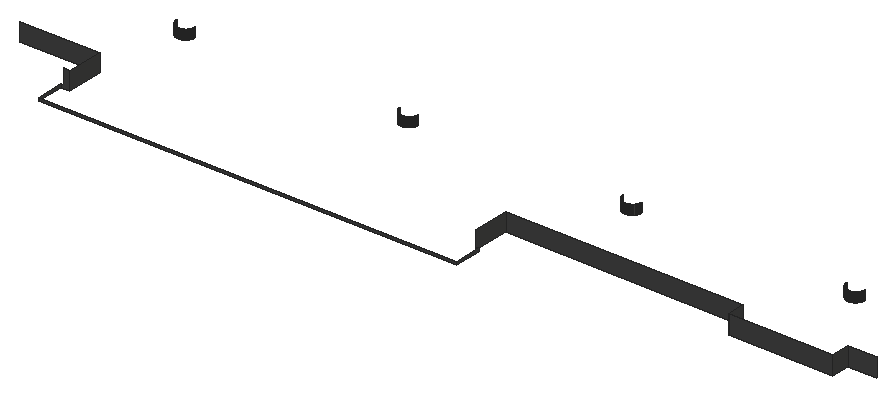
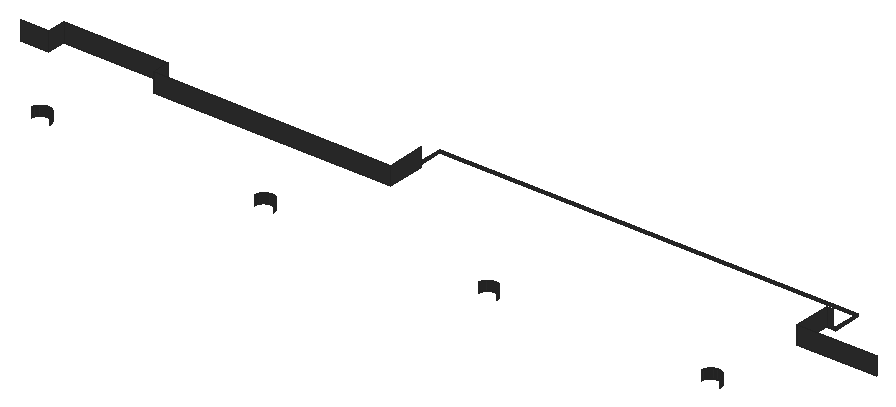
# SketchUp Ruby script. Lengths in inches.
U = 1.inch
M = Sketchup.active_model
def pt(a) = Geom::Point3d.new(a.map { |v| v * U })
def face(e, loops, mat)
  f = e.add_face(loops[0].map { |a| pt(a) })
  loops[1..].each { |l| e.add_face(l.map { |a| pt(a) }).erase! }
  f.material = f.back_material = mat if mat
  f
end
# faces: each face lists its corners as indices into pts; further lists are holes
def faces(e, pts, list, mat = nil) = list.each { |f| face(e, (f[0].is_a?(Array) ? f : [f]).map { |l| l.map { |i| pts[i] } }, mat) }
# xy, xz, yz: faces in a plane at the given z, y or x. An outline is a flat list of corners, or four numbers for a rectangle; further outlines are holes
def ring(l) = l.size == 4 ? [[l[0], l[1]], [l[2], l[1]], [l[2], l[3]], [l[0], l[3]]] : l.each_slice(2).to_a
def flat(e, list, mat, &to3) = list.each { |f| face(e, (f[0].is_a?(Array) ? f : [f]).map { |l| ring(l).map { |u, v| to3.(u, v) } }, mat) }
def xy(e, z, list, mat = nil) = flat(e, list, mat) { |x, y| [x, y, z] }
def xz(e, y, list, mat = nil) = flat(e, list, mat) { |x, z| [x, y, z] }
def yz(e, x, list, mat = nil) = flat(e, list, mat) { |y, z| [x, y, z] }
def lines(e, pts, list) = list.each { |a, b| e.add_line(pt(pts[a]), pt(pts[b])) }
# prism: a flat outline (further loops are holes) pulled along v
def prism(e, loops, v, mat = nil)
  f = face(e, loops, mat); d = Geom::Vector3d.new(v.map { |x| x * U })
  f.pushpull(f.normal.samedirection?(d) ? d.length : -d.length)
end
def box(e, o, s, mat = nil) = prism(e, [[o, [o[0] + s[0], o[1], o[2]], [o[0] + s[0], o[1] + s[1], o[2]], [o[0], o[1] + s[1], o[2]]]], [0, 0, s[2]], mat)
def at(x, y, z, deg = 0) = Geom::Transformation.translation(pt([x, y, z])) * Geom::Transformation.rotation(ORIGIN, Z_AXIS, deg.degrees)
def axes(o, x, y, z) = Geom::Transformation.new([*x, 0, *y, 0, *z, 0, *pt(o).to_a, 1])
def part(name) = M.definitions.add(name)
# library, detail: a bought-in or finely detailed component or shape, given as its bounding box
def library(name, o, s) = part(name).tap { |d| box(d.entities, o, s) }
def detail(e, o, s) = box(e.add_group.entities, o, s)
def put(e, d, t, mat = nil) = e.add_instance(d, t).tap { |i| i.material = mat if mat }
def group(e, t, mat = nil) = e.add_group.tap { |g| g.transformation = t; g.material = mat if mat }.entities
root = M.entities
M.materials.add("1448 AP 8253 RAVEN SONG").color = [64, 64, 63]
xz(root,174,[[31.93,372,167.89,373]],"1448 AP 8253 RAVEN SONG")
xz(root,183,[[31.93,372,31.93,373,32.96,373,32.96,378,35.02,378,35.02,372],[166.86,372,167.89,373]],"1448 AP 8253 RAVEN SONG")
xz(root,189,[[244.11,372,278.1,378]],"1448 AP 8253 RAVEN SONG")
xz(root,195,[[9.27,372,35.02,378],[166.86,372,244.11,378],[278.1,372,287.37,378]],"1448 AP 8253 RAVEN SONG")
xz(root,221.5,[[39.29,372,39.37,375],[39.37,372,39.45,375],[39.45,372,39.53,375],[39.53,372,39.61,375],[111.87,372,111.95,375],
  [111.95,372,112.03,375],[112.03,372,112.11,375],[112.11,372,112.1875,375],[184.45,372,184.53,375],[184.53,372,184.61,375],
  [184.61,372,184.6875,375],[184.6875,372,184.77,375],[257.03,372,257.11,375],[257.11,372,257.19,375],[257.19,372,257.27,375],
  [257.27,372,257.35,375]],"1448 AP 8253 RAVEN SONG")
yz(root,31.93,[[174,372,183,373]],"1448 AP 8253 RAVEN SONG")
yz(root,35.02,[[183,372,195,378]],"1448 AP 8253 RAVEN SONG")
yz(root,36.45,[[224.34,372,224.42,375]],"1448 AP 8253 RAVEN SONG")
yz(root,42.45,[[224.34,372,224.42,375]],"1448 AP 8253 RAVEN SONG")
yz(root,109.03,[[224.34,372,224.42,375]],"1448 AP 8253 RAVEN SONG")
yz(root,115.03,[[224.34,372,224.42,375]],"1448 AP 8253 RAVEN SONG")
yz(root,166.86,[[183,372,195,378]],"1448 AP 8253 RAVEN SONG")
yz(root,167.89,[[174,372,183,373]],"1448 AP 8253 RAVEN SONG")
yz(root,181.61,[[224.34,372,224.42,375]],"1448 AP 8253 RAVEN SONG")
yz(root,187.61,[[224.34,372,224.42,375],[224.42,372,224.5,375]],"1448 AP 8253 RAVEN SONG")
yz(root,244.11,[[189,372,195,378]],"1448 AP 8253 RAVEN SONG")
yz(root,254.19,[[224.34,372,224.42,375],[224.42,372,224.5,375]],"1448 AP 8253 RAVEN SONG")
yz(root,260.1875,[[224.34,372,224.42,375]],"1448 AP 8253 RAVEN SONG")
yz(root,278.1,[[189,372,195,378]],"1448 AP 8253 RAVEN SONG")
p = [[38.98,221.54,372],[38.9,221.55,372],[38.9,221.55,375],[38.98,221.54,375],[39.06,221.53,372],[39.06,221.53,375],
  [39.21,221.51,372],[39.14,221.52,372],[39.14,221.52,375],[39.21,221.51,375],[39.29,221.5,372],[39.29,221.5,375],
  [39.69,221.51,372],[39.61,221.5,372],[39.61,221.5,375],[39.69,221.51,375],[39.76,221.52,372],[39.76,221.52,375],
  [39.84,221.53,372],[39.84,221.53,375],[39.92,221.54,372],[39.92,221.54,375],[40,221.55,372],[40,221.55,375],
  [111.5625,221.54,372],[111.48,221.55,372],[111.48,221.55,375],[111.5625,221.54,375],[111.72,221.52,372],[111.64,221.53,372],
  [111.64,221.53,375],[111.72,221.52,375],[111.79,221.51,372],[111.79,221.51,375],[111.87,221.5,372],[111.87,221.5,375],
  [112.27,221.51,372],[112.1875,221.5,372],[112.1875,221.5,375],[112.27,221.51,375],[112.34,221.52,372],[112.34,221.52,375],
  [112.42,221.53,372],[112.42,221.53,375],[112.5,221.54,372],[112.5,221.54,375],[112.58,221.55,372],[112.58,221.55,375],
  [184.22,221.53,372],[184.14,221.54,372],[184.14,221.54,375],[184.22,221.53,375],[184.0625,221.55,372],[184.0625,221.55,375],
  [184.3,221.52,372],[184.3,221.52,375],[184.375,221.51,372],[184.375,221.51,375],[184.45,221.5,372],[184.45,221.5,375],
  [184.85,221.51,372],[184.77,221.5,372],[184.77,221.5,375],[184.85,221.51,375],[184.92,221.52,372],[184.92,221.52,375],
  [185,221.53,372],[185,221.53,375],[185.08,221.54,372],[185.08,221.54,375],[185.16,221.55,372],[185.16,221.55,375],
  [256.72,221.54,372],[256.64,221.55,372],[256.64,221.55,375],[256.72,221.54,375],[256.8,221.53,372],[256.8,221.53,375],
  [256.875,221.52,372],[256.875,221.52,375],[256.95,221.51,372],[256.95,221.51,375],[257.03,221.5,372],[257.03,221.5,375],
  [257.43,221.51,372],[257.35,221.5,372],[257.35,221.5,375],[257.43,221.51,375],[257.5,221.52,372],[257.5,221.52,375],
  [257.58,221.53,372],[257.58,221.53,375],[257.66,221.54,372],[257.66,221.54,375],[257.74,221.55,372],[257.74,221.55,375],
  [38.52,221.65,372],[38.45,221.67,372],[38.45,221.67,375],[38.52,221.65,375],[38.6,221.625,372],[38.6,221.625,375],
  [38.67,221.6,372],[38.67,221.6,375],[38.83,221.57,372],[38.75,221.58,372],[38.75,221.58,375],[38.83,221.57,375],
  [40.07,221.57,372],[40.07,221.57,375],[40.15,221.58,372],[40.15,221.58,375],[40.23,221.6,372],[40.23,221.6,375],
  [40.3,221.625,372],[40.3,221.625,375],[40.38,221.65,372],[40.38,221.65,375],[40.45,221.67,372],[40.45,221.67,375],
  [111.1,221.65,372],[111.03,221.67,372],[111.03,221.67,375],[111.1,221.65,375],[111.18,221.625,372],[111.18,221.625,375],
  [111.25,221.6,372],[111.25,221.6,375],[111.41,221.57,372],[111.33,221.58,372],[111.33,221.58,375],[111.41,221.57,375],
  [112.65,221.57,372],[112.65,221.57,375],[112.73,221.58,372],[112.73,221.58,375],[112.81,221.6,372],[112.81,221.6,375],
  [112.88,221.625,372],[112.88,221.625,375],[112.96,221.65,372],[112.96,221.65,375],[113.03,221.67,372],[113.03,221.67,375],
  [183.68,221.65,372],[183.61,221.67,372],[183.61,221.67,375],[183.68,221.65,375],[183.76,221.625,372],[183.76,221.625,375],
  [183.91,221.58,372],[183.83,221.6,372],[183.83,221.6,375],[183.91,221.58,375],[183.99,221.57,372],[183.99,221.57,375],
  [185.23,221.57,372],[185.23,221.57,375],[185.31,221.58,372],[185.31,221.58,375],[185.39,221.6,372],[185.39,221.6,375],
  [185.46,221.625,372],[185.46,221.625,375],[185.54,221.65,372],[185.54,221.65,375],[185.61,221.67,372],[185.61,221.67,375],
  [256.26,221.65,372],[256.1875,221.67,372],[256.1875,221.67,375],[256.26,221.65,375],[256.41,221.6,372],[256.34,221.625,372],
  [256.34,221.625,375],[256.41,221.6,375],[256.49,221.58,372],[256.49,221.58,375],[256.57,221.57,372],[256.57,221.57,375],
  [257.8125,221.57,372],[257.8125,221.57,375],[257.89,221.58,372],[257.89,221.58,375],[257.97,221.6,372],[257.97,221.6,375],
  [258.04,221.625,372],[258.04,221.625,375],[258.12,221.65,372],[258.12,221.65,375],[258.19,221.67,372],[258.19,221.67,375],
  [38.3,221.73,372],[38.23,221.76,372],[38.23,221.76,375],[38.3,221.73,375],[38.375,221.7,372],[38.375,221.7,375],
  [40.53,221.7,372],[40.53,221.7,375],[40.6,221.73,372],[40.6,221.73,375],[40.67,221.76,372],[40.67,221.76,375],
  [110.88,221.73,372],[110.81,221.76,372],[110.81,221.76,375],[110.88,221.73,375],[110.95,221.7,372],[110.95,221.7,375],
  [113.11,221.7,372],[113.11,221.7,375],[113.18,221.73,372],[113.18,221.73,375],[113.25,221.76,372],[113.25,221.76,375],
  [183.46,221.73,372],[183.39,221.76,372],[183.39,221.76,375],[183.46,221.73,375],[183.53,221.7,372],[183.53,221.7,375],
  [185.69,221.7,372],[185.69,221.7,375],[185.76,221.73,372],[185.76,221.73,375],[185.83,221.76,372],[185.83,221.76,375],
  [256.11,221.7,372],[256.04,221.73,372],[256.04,221.73,375],[256.11,221.7,375],[255.97,221.76,372],[255.97,221.76,375],
  [258.27,221.7,372],[258.27,221.7,375],[258.34,221.73,372],[258.34,221.73,375],[258.41,221.76,372],[258.41,221.76,375],
  [38.09,221.83,372],[38.02,221.86,372],[38.02,221.86,375],[38.09,221.83,375],[38.16,221.79,372],[38.16,221.79,375],
  [40.74,221.79,372],[40.74,221.79,375],[40.8125,221.83,372],[40.8125,221.83,375],[40.88,221.86,372],[40.88,221.86,375],
  [110.67,221.83,372],[110.6,221.86,372],[110.6,221.86,375],[110.67,221.83,375],[110.74,221.79,372],[110.74,221.79,375],
  [113.32,221.79,372],[113.32,221.79,375],[113.39,221.83,372],[113.39,221.83,375],[113.46,221.86,372],[113.46,221.86,375],
  [183.32,221.79,372],[183.25,221.83,372],[183.25,221.83,375],[183.32,221.79,375],[183.18,221.86,372],[183.18,221.86,375],
  [185.9,221.79,372],[185.9,221.79,375],[185.97,221.83,372],[185.97,221.83,375],[186.04,221.86,372],[186.04,221.86,375],
  [255.9,221.79,372],[255.83,221.83,372],[255.83,221.83,375],[255.9,221.79,375],[255.76,221.86,372],[255.76,221.86,375],
  [258.48,221.79,372],[258.48,221.79,375],[258.55,221.83,372],[258.55,221.83,375],[258.62,221.86,372],[258.62,221.86,375],
  [37.88,221.94,372],[37.82,221.98,372],[37.82,221.98,375],[37.88,221.94,375],[37.95,221.9,372],[37.95,221.9,375],
  [40.95,221.9,372],[40.95,221.9,375],[41.02,221.94,372],[41.02,221.94,375],[41.08,221.98,372],[41.08,221.98,375],
  [110.46,221.94,372],[110.4,221.98,372],[110.4,221.98,375],[110.46,221.94,375],[110.53,221.9,372],[110.53,221.9,375],
  [113.53,221.9,372],[113.53,221.9,375],[113.6,221.94,372],[113.6,221.94,375],[113.66,221.98,372],[113.66,221.98,375],
  [183.11,221.9,372],[183.04,221.94,372],[183.04,221.94,375],[183.11,221.9,375],[182.98,221.98,372],[182.98,221.98,375],
  [186.11,221.9,372],[186.11,221.9,375],[186.18,221.94,372],[186.18,221.94,375],[186.24,221.98,372],[186.24,221.98,375],
  [255.69,221.9,372],[255.62,221.94,372],[255.62,221.94,375],[255.69,221.9,375],[255.56,221.98,372],[255.56,221.98,375],
  [258.69,221.9,372],[258.69,221.9,375],[258.76,221.94,372],[258.76,221.94,375],[258.82,221.98,372],[258.82,221.98,375],
  [37.75,222.03,372],[37.6875,222.07,372],[37.6875,222.07,375],[37.75,222.03,375],[41.15,222.03,372],[41.15,222.03,375],
  [41.21,222.07,372],[41.21,222.07,375],[110.33,222.03,372],[110.33,222.03,375],[110.27,222.07,372],[110.27,222.07,375],
  [113.73,222.03,372],[113.73,222.03,375],[113.79,222.07,372],[113.79,222.07,375],[182.91,222.03,372],[182.85,222.07,372],
  [182.85,222.07,375],[182.91,222.03,375],[186.31,222.03,372],[186.31,222.03,375],[186.375,222.07,372],[186.375,222.07,375],
  [255.49,222.03,372],[255.43,222.07,372],[255.43,222.07,375],[255.49,222.03,375],[258.89,222.03,372],[258.89,222.03,375],
  [258.95,222.07,372],[258.95,222.07,375],[37.625,222.12,372],[37.625,222.12,375],[37.5625,222.17,372],[37.5625,222.17,375],
  [41.28,222.12,372],[41.28,222.12,375],[41.34,222.17,372],[41.34,222.17,375],[110.2,222.12,372],[110.14,222.17,372],
  [110.14,222.17,375],[110.2,222.12,375],[113.86,222.12,372],[113.86,222.12,375],[113.92,222.17,372],[113.92,222.17,375],
  [182.78,222.12,372],[182.72,222.17,372],[182.72,222.17,375],[182.78,222.12,375],[186.4375,222.12,372],[186.4375,222.12,375],
  [186.5,222.17,372],[186.5,222.17,375],[255.36,222.12,372],[255.3,222.17,372],[255.3,222.17,375],[255.36,222.12,375],
  [259.02,222.12,372],[259.02,222.12,375],[259.08,222.17,372],[259.08,222.17,375],[37.5,222.22,372],[37.44,222.27,372],
  [37.44,222.27,375],[37.5,222.22,375],[41.4,222.22,372],[41.4,222.22,375],[41.46,222.27,372],[41.46,222.27,375],
  [110.08,222.22,372],[110.02,222.27,372],[110.02,222.27,375],[110.08,222.22,375],[113.98,222.22,372],[113.98,222.22,375],
  [114.04,222.27,372],[114.04,222.27,375],[182.66,222.22,372],[182.6,222.27,372],[182.6,222.27,375],[182.66,222.22,375],
  [186.56,222.22,372],[186.56,222.22,375],[186.62,222.27,372],[186.62,222.27,375],[255.24,222.22,372],[255.24,222.22,375],
  [255.18,222.27,372],[255.18,222.27,375],[259.14,222.22,372],[259.14,222.22,375],[259.2,222.27,372],[259.2,222.27,375],
  [37.38,222.32,372],[37.33,222.38,372],[37.33,222.38,375],[37.38,222.32,375],[41.52,222.32,372],[41.52,222.32,375],
  [41.57,222.38,372],[41.57,222.38,375],[109.96,222.32,372],[109.91,222.38,372],[109.91,222.38,375],[109.96,222.32,375],
  [114.1,222.32,372],[114.1,222.32,375],[114.15,222.38,372],[114.15,222.38,375],[182.54,222.32,372],[182.54,222.32,375],
  [182.49,222.38,372],[182.49,222.38,375],[186.68,222.32,372],[186.68,222.32,375],[186.73,222.38,372],[186.73,222.38,375],
  [255.125,222.32,372],[255.125,222.32,375],[255.07,222.38,372],[255.07,222.38,375],[259.26,222.32,372],[259.26,222.32,375],
  [259.3125,222.38,372],[259.3125,222.38,375],[37.27,222.43,372],[37.22,222.49,372],[37.22,222.49,375],[37.27,222.43,375],
  [41.625,222.43,372],[41.625,222.43,375],[41.68,222.49,372],[41.68,222.49,375],[109.85,222.43,372],[109.8,222.49,372],
  [109.8,222.49,375],[109.85,222.43,375],[114.21,222.43,372],[114.21,222.43,375],[114.26,222.49,372],[114.26,222.49,375],
  [182.43,222.43,372],[182.43,222.43,375],[182.38,222.49,372],[182.38,222.49,375],[186.79,222.43,372],[186.79,222.43,375],
  [186.84,222.49,372],[186.84,222.49,375],[255.01,222.43,372],[255.01,222.43,375],[254.96,222.49,372],[254.96,222.49,375],
  [259.37,222.43,372],[259.37,222.43,375],[259.42,222.49,372],[259.42,222.49,375],[37.17,222.55,372],[37.17,222.55,375],
  [41.73,222.55,372],[41.73,222.55,375],[109.75,222.55,372],[109.75,222.55,375],[114.3125,222.55,372],[114.3125,222.55,375],
  [182.33,222.55,372],[182.33,222.55,375],[186.89,222.55,372],[186.89,222.55,375],[254.91,222.55,372],[254.91,222.55,375],
  [259.47,222.55,372],[259.47,222.55,375],[37.12,222.61,372],[37.12,222.61,375],[37.07,222.67,372],[37.07,222.67,375],
  [41.78,222.61,372],[41.78,222.61,375],[41.83,222.67,372],[41.83,222.67,375],[109.7,222.61,372],[109.65,222.67,372],
  [109.65,222.67,375],[109.7,222.61,375],[114.36,222.61,372],[114.36,222.61,375],[114.41,222.67,372],[114.41,222.67,375],
  [182.28,222.61,372],[182.23,222.67,372],[182.23,222.67,375],[182.28,222.61,375],[186.94,222.61,372],[186.94,222.61,375],
  [186.99,222.67,372],[186.99,222.67,375],[254.86,222.61,372],[254.81,222.67,372],[254.81,222.67,375],[254.86,222.61,375],
  [259.52,222.61,372],[259.52,222.61,375],[259.57,222.67,372],[259.57,222.67,375],[37.02,222.74,372],[37.02,222.74,375],
  [36.98,222.8,372],[36.98,222.8,375],[41.88,222.74,372],[41.88,222.74,375],[41.92,222.8,372],[41.92,222.8,375],
  [109.6,222.74,372],[109.6,222.74,375],[109.56,222.8,372],[109.56,222.8,375],[114.46,222.74,372],[114.46,222.74,375],
  [114.5,222.8,372],[114.5,222.8,375],[182.18,222.74,372],[182.14,222.8,372],[182.14,222.8,375],[182.18,222.74,375],
  [187.04,222.74,372],[187.04,222.74,375],[187.08,222.8,372],[187.08,222.8,375],[254.76,222.74,372],[254.72,222.8,372],
  [254.72,222.8,375],[254.76,222.74,375],[259.62,222.74,372],[259.62,222.74,375],[259.66,222.8,372],[259.66,222.8,375],
  [36.93,222.87,372],[36.93,222.87,375],[41.97,222.87,372],[41.97,222.87,375],[109.51,222.87,372],[109.51,222.87,375],
  [114.55,222.87,372],[114.55,222.87,375],[182.09,222.87,372],[182.09,222.87,375],[187.125,222.87,372],[187.125,222.87,375],
  [254.67,222.87,372],[254.67,222.87,375],[259.71,222.87,372],[259.71,222.87,375],[36.89,222.93,372],[36.89,222.93,375],
  [36.85,223,372],[36.85,223,375],[42.01,222.93,372],[42.01,222.93,375],[42.05,223,372],[42.05,223,375],
  [109.47,222.93,372],[109.43,223,372],[109.43,223,375],[109.47,222.93,375],[114.59,222.93,372],[114.59,222.93,375],
  [114.63,223,372],[114.63,223,375],[182.05,222.93,372],[182.01,223,372],[182.01,223,375],[182.05,222.93,375],
  [187.17,222.93,372],[187.17,222.93,375],[187.21,223,372],[187.21,223,375],[254.63,222.93,372],[254.63,222.93,375],
  [254.59,223,372],[254.59,223,375],[259.75,222.93,372],[259.75,222.93,375],[259.79,223,372],[259.79,223,375],
  [36.8125,223.07,372],[36.8125,223.07,375],[42.09,223.07,372],[42.09,223.07,375],[109.39,223.07,372],[109.39,223.07,375],
  [114.67,223.07,372],[114.67,223.07,375],[181.97,223.07,372],[181.97,223.07,375],[187.25,223.07,372],[187.25,223.07,375],
  [254.55,223.07,372],[254.55,223.07,375],[259.83,223.07,372],[259.83,223.07,375],[36.78,223.14,372],[36.74,223.21,372],
  [36.74,223.21,375],[36.78,223.14,375],[42.125,223.14,372],[42.125,223.14,375],[42.16,223.21,372],[42.16,223.21,375],
  [109.36,223.14,372],[109.32,223.21,372],[109.32,223.21,375],[109.36,223.14,375],[114.7,223.14,372],[114.7,223.14,375],
  [114.74,223.21,372],[114.74,223.21,375],[181.9375,223.14,372],[181.9375,223.14,375],[181.9,223.21,372],[181.9,223.21,375],
  [187.28,223.14,372],[187.28,223.14,375],[187.32,223.21,372],[187.32,223.21,375],[254.52,223.14,372],[254.52,223.14,375],
  [254.48,223.21,372],[254.48,223.21,375],[259.86,223.14,372],[259.86,223.14,375],[259.9,223.21,372],[259.9,223.21,375],
  [36.71,223.28,372],[36.71,223.28,375],[42.19,223.28,372],[42.19,223.28,375],[109.29,223.28,372],[109.29,223.28,375],
  [114.77,223.28,372],[114.77,223.28,375],[181.87,223.28,372],[181.87,223.28,375],[187.35,223.28,372],[187.35,223.28,375],
  [254.45,223.28,372],[254.45,223.28,375],[259.93,223.28,372],[259.93,223.28,375],[36.68,223.35,372],[36.68,223.35,375],
  [42.22,223.35,372],[42.22,223.35,375],[109.26,223.35,372],[109.26,223.35,375],[114.8,223.35,372],[114.8,223.35,375],
  [181.84,223.35,372],[181.84,223.35,375],[187.38,223.35,372],[187.38,223.35,375],[254.42,223.35,372],[254.42,223.35,375],
  [259.96,223.35,372],[259.96,223.35,375],[36.65,223.42,372],[36.65,223.42,375],[36.62,223.5,372],[36.62,223.5,375],
  [42.25,223.42,372],[42.25,223.42,375],[42.28,223.5,372],[42.28,223.5,375],[109.23,223.42,372],[109.23,223.42,375],
  [109.2,223.5,372],[109.2,223.5,375],[114.83,223.42,372],[114.83,223.42,375],[114.86,223.5,372],[114.86,223.5,375],
  [181.81,223.42,372],[181.81,223.42,375],[181.78,223.5,372],[181.78,223.5,375],[187.41,223.42,372],[187.41,223.42,375],
  [187.4375,223.5,372],[187.4375,223.5,375],[254.39,223.42,372],[254.39,223.42,375],[254.36,223.5,372],[254.36,223.5,375],
  [259.99,223.42,372],[259.99,223.42,375],[260.02,223.5,372],[260.02,223.5,375],[36.6,223.57,372],[36.6,223.57,375],
  [42.3,223.57,372],[42.3,223.57,375],[109.18,223.57,372],[109.18,223.57,375],[114.88,223.57,372],[114.88,223.57,375],
  [181.76,223.57,372],[181.76,223.57,375],[187.46,223.57,372],[187.46,223.57,375],[254.34,223.57,372],[254.34,223.57,375],
  [260.04,223.57,372],[260.04,223.57,375],[36.57,223.65,372],[36.57,223.65,375],[36.55,223.72,372],[36.55,223.72,375],
  [42.33,223.65,372],[42.33,223.65,375],[42.35,223.72,372],[42.35,223.72,375],[109.15,223.65,372],[109.13,223.72,372],
  [109.13,223.72,375],[109.15,223.65,375],[114.91,223.65,372],[114.91,223.65,375],[114.93,223.72,372],[114.93,223.72,375],
  [181.73,223.65,372],[181.73,223.65,375],[181.71,223.72,372],[181.71,223.72,375],[187.49,223.65,372],[187.49,223.65,375],
  [187.51,223.72,372],[187.51,223.72,375],[254.3125,223.65,372],[254.3125,223.65,375],[254.29,223.72,372],[254.29,223.72,375],
  [260.07,223.65,372],[260.07,223.65,375],[260.09,223.72,372],[260.09,223.72,375],[36.53,223.8,372],[36.53,223.8,375],
  [42.37,223.8,372],[42.37,223.8,375],[109.11,223.8,372],[109.11,223.8,375],[114.95,223.8,372],[114.95,223.8,375],
  [181.69,223.8,372],[181.69,223.8,375],[187.53,223.8,372],[187.53,223.8,375],[254.27,223.8,372],[254.27,223.8,375],
  [260.11,223.8,372],[260.11,223.8,375],[36.52,223.875,372],[36.52,223.875,375],[42.38,223.875,372],[42.38,223.875,375],
  [109.1,223.875,372],[109.1,223.875,375],[114.96,223.875,372],[114.96,223.875,375],[181.68,223.875,372],[181.68,223.875,375],
  [187.54,223.875,372],[187.54,223.875,375],[254.26,223.875,372],[254.26,223.875,375],[260.125,223.875,372],[260.125,223.875,375],
  [36.5,223.95,372],[36.5,223.95,375],[42.4,223.95,372],[42.4,223.95,375],[109.08,223.95,372],[109.08,223.95,375],
  [114.98,223.95,372],[114.98,223.95,375],[181.66,223.95,372],[181.66,223.95,375],[187.56,223.95,372],[187.56,223.95,375],
  [254.24,223.95,372],[254.24,223.95,375],[260.14,223.95,372],[260.14,223.95,375],[36.49,224.03,372],[36.49,224.03,375],
  [36.48,224.11,372],[36.48,224.11,375],[42.41,224.03,372],[42.41,224.03,375],[42.42,224.11,372],[42.42,224.11,375],
  [109.07,224.03,372],[109.07,224.03,375],[109.06,224.11,372],[109.06,224.11,375],[114.99,224.03,372],[114.99,224.03,375],
  [115,224.11,372],[115,224.11,375],[181.65,224.03,372],[181.65,224.03,375],[181.64,224.11,372],[181.64,224.11,375],
  [187.57,224.03,372],[187.57,224.03,375],[187.58,224.11,372],[187.58,224.11,375],[254.23,224.03,372],[254.23,224.03,375],
  [254.22,224.11,372],[254.22,224.11,375],[260.15,224.03,372],[260.15,224.03,375],[260.16,224.11,372],[260.16,224.11,375],
  [36.47,224.1875,372],[36.47,224.1875,375],[42.43,224.1875,372],[42.43,224.1875,375],[109.05,224.1875,372],[109.05,224.1875,375],
  [115.01,224.1875,372],[115.01,224.1875,375],[181.625,224.1875,372],[181.625,224.1875,375],[187.59,224.1875,372],[187.59,224.1875,375],
  [254.21,224.1875,372],[254.21,224.1875,375],[260.17,224.1875,372],[260.17,224.1875,375],[36.46,224.26,372],[36.46,224.26,375],
  [42.44,224.26,372],[42.44,224.26,375],[109.04,224.26,372],[109.04,224.26,375],[115.02,224.26,372],[115.02,224.26,375],
  [181.62,224.26,372],[181.62,224.26,375],[187.6,224.26,372],[187.6,224.26,375],[254.2,224.26,372],[254.2,224.26,375],
  [260.18,224.26,372],[260.18,224.26,375],[36.45,224.34,372],[36.45,224.34,375],[42.45,224.34,372],[42.45,224.34,375],
  [109.03,224.34,372],[109.03,224.34,375],[115.03,224.34,372],[115.03,224.34,375],[181.61,224.34,372],[181.61,224.34,375],
  [187.61,224.34,372],[187.61,224.34,375],[254.19,224.34,372],[254.19,224.34,375],[260.1875,224.34,372],[260.1875,224.34,375],
  [260.19,224.5,372],[260.1875,224.42,372],[260.1875,224.42,375],[260.19,224.5,375]]
faces(root,p,[[0,1,2,3],[4,0,3,5],[6,7,8,9],[7,4,5,8],[10,6,9,11],[12,13,14,15],[16,12,15,17],[18,16,17,19],
  [20,18,19,21],[22,20,21,23],[24,25,26,27],[28,29,30,31],[29,24,27,30],[32,28,31,33],[34,32,33,35],[36,37,38,39],
  [40,36,39,41],[42,40,41,43],[44,42,43,45],[46,44,45,47],[48,49,50,51],[49,52,53,50],[54,48,51,55],[56,54,55,57],
  [58,56,57,59],[60,61,62,63],[64,60,63,65],[66,64,65,67],[68,66,67,69],[70,68,69,71],[72,73,74,75],[76,72,75,77],
  [78,76,77,79],[80,78,79,81],[82,80,81,83],[84,85,86,87],[88,84,87,89],[90,88,89,91],[92,90,91,93],[94,92,93,95],
  [96,97,98,99],[100,96,99,101],[102,100,101,103],[104,105,106,107],[105,102,103,106],[1,104,107,2],[108,22,23,109],[110,108,109,111],
  [112,110,111,113],[114,112,113,115],[116,114,115,117],[118,116,117,119],[120,121,122,123],[124,120,123,125],[126,124,125,127],[128,129,130,131],
  [129,126,127,130],[25,128,131,26],[132,46,47,133],[134,132,133,135],[136,134,135,137],[138,136,137,139],[140,138,139,141],[142,140,141,143],
  [144,145,146,147],[148,144,147,149],[150,151,152,153],[151,148,149,152],[154,150,153,155],[52,154,155,53],[156,70,71,157],[158,156,157,159],
  [160,158,159,161],[162,160,161,163],[164,162,163,165],[166,164,165,167],[168,169,170,171],[172,173,174,175],[173,168,171,174],[176,172,175,177],
  [178,176,177,179],[73,178,179,74],[180,94,95,181],[182,180,181,183],[184,182,183,185],[186,184,185,187],[188,186,187,189],[190,188,189,191],
  [192,193,194,195],[196,192,195,197],[97,196,197,98],[198,118,119,199],[200,198,199,201],[202,200,201,203],[204,205,206,207],[208,204,207,209],
  [121,208,209,122],[210,142,143,211],[212,210,211,213],[214,212,213,215],[216,217,218,219],[145,220,221,146],[220,216,219,221],[222,166,167,223],
  [224,222,223,225],[226,224,225,227],[228,229,230,231],[229,232,233,230],[169,228,231,170],[234,190,191,235],[236,234,235,237],[238,236,237,239],
  [240,241,242,243],[244,240,243,245],[193,244,245,194],[246,202,203,247],[248,246,247,249],[250,248,249,251],[252,253,254,255],[205,256,257,206],
  [256,252,255,257],[258,214,215,259],[260,258,259,261],[262,260,261,263],[264,265,266,267],[265,268,269,266],[217,264,267,218],[270,226,227,271],
  [272,270,271,273],[274,272,273,275],[276,277,278,279],[277,280,281,278],[232,276,279,233],[282,238,239,283],[284,282,283,285],[286,284,285,287],
  [288,289,290,291],[241,292,293,242],[292,288,291,293],[294,250,251,295],[296,294,295,297],[298,296,297,299],[300,301,302,303],[253,304,305,254],
  [304,300,303,305],[306,262,263,307],[308,306,307,309],[310,308,309,311],[312,313,314,315],[313,316,317,314],[268,312,315,269],[318,274,275,319],
  [320,318,319,321],[322,320,321,323],[324,325,326,327],[325,328,329,326],[280,324,327,281],[330,286,287,331],[332,330,331,333],[334,332,333,335],
  [336,337,338,339],[289,336,339,290],[340,298,299,341],[342,340,341,343],[301,344,345,302],[344,346,347,345],[348,310,311,349],[350,348,349,351],
  [352,353,354,355],[316,352,355,317],[356,322,323,357],[358,356,357,359],[360,361,362,363],[328,360,363,329],[364,334,335,365],[366,364,365,367],
  [337,368,369,338],[368,370,371,369],[372,342,343,373],[374,372,373,375],[376,377,378,379],[346,376,379,347],[380,350,351,381],[382,380,381,383],
  [384,385,386,387],[353,384,387,354],[388,358,359,389],[390,388,389,391],[392,393,394,395],[361,392,395,362],[396,366,367,397],[398,396,397,399],
  [400,401,402,403],[370,400,403,371],[404,374,375,405],[406,404,405,407],[408,409,410,411],[377,408,411,378],[412,382,383,413],[414,412,413,415],
  [416,417,418,419],[385,416,419,386],[420,390,391,421],[422,420,421,423],[393,424,425,394],[424,426,427,425],[428,398,399,429],[430,428,429,431],
  [432,433,434,435],[401,432,435,402],[436,406,407,437],[438,436,437,439],[440,441,442,443],[409,440,443,410],[444,414,415,445],[446,444,445,447],
  [417,448,449,418],[448,450,451,449],[452,422,423,453],[454,452,453,455],[426,456,457,427],[456,458,459,457],[460,430,431,461],[462,460,461,463],
  [464,465,466,467],[433,464,467,434],[468,438,439,469],[470,468,469,471],[472,473,474,475],[441,472,475,442],[476,446,447,477],[478,476,477,479],
  [450,480,481,451],[480,482,483,481],[484,454,455,485],[486,484,485,487],[458,488,489,459],[488,490,491,489],[492,462,463,493],[494,492,493,495],
  [465,496,497,466],[498,470,471,499],[473,500,501,474],[502,478,479,503],[482,504,505,483],[506,486,487,507],[490,508,509,491],[510,494,495,511],
  [496,512,513,497],[512,514,515,513],[516,498,499,517],[518,516,517,519],[520,521,522,523],[500,520,523,501],[524,502,503,525],[526,524,525,527],
  [528,529,530,531],[504,528,531,505],[532,506,507,533],[534,532,533,535],[536,537,538,539],[508,536,539,509],[540,510,511,541],[542,540,541,543],
  [514,544,545,515],[544,546,547,545],[548,518,519,549],[550,548,549,551],[521,552,553,522],[552,554,555,553],[556,526,527,557],[558,556,557,559],
  [560,561,562,563],[529,560,563,530],[564,534,535,565],[566,564,565,567],[568,569,570,571],[537,568,571,538],[572,542,543,573],[574,572,573,575],
  [546,576,577,547],[578,550,551,579],[554,580,581,555],[582,558,559,583],[561,584,585,562],[586,566,567,587],[569,588,589,570],[590,574,575,591],
  [576,592,593,577],[592,594,595,593],[596,578,579,597],[598,596,597,599],[600,601,602,603],[580,600,603,581],[604,582,583,605],[606,604,605,607],
  [608,609,610,611],[584,608,611,585],[612,586,587,613],[614,612,613,615],[588,616,617,589],[616,618,619,617],[620,590,591,621],[622,620,621,623],
  [594,624,625,595],[626,598,599,627],[601,628,629,602],[630,606,607,631],[609,632,633,610],[634,614,615,635],[618,636,637,619],[638,622,623,639],
  [640,641,642,643],[624,640,643,625],[644,626,627,645],[646,644,645,647],[648,649,650,651],[628,648,651,629],[652,630,631,653],[654,652,653,655],
  [632,656,657,633],[656,658,659,657],[660,634,635,661],[662,660,661,663],[636,664,665,637],[664,666,667,665],[668,638,639,669],[670,668,669,671],
  [641,672,673,642],[674,646,647,675],[649,676,677,650],[678,654,655,679],[658,680,681,659],[682,662,663,683],[666,684,685,667],[686,670,671,687],
  [672,688,689,673],[690,674,675,691],[676,692,693,677],[694,678,679,695],[680,696,697,681],[698,682,683,699],[684,700,701,685],[702,686,687,703],
  [688,704,705,689],[704,706,707,705],[708,690,691,709],[710,708,709,711],[692,712,713,693],[712,714,715,713],[716,694,695,717],[718,716,717,719],
  [696,720,721,697],[720,722,723,721],[724,698,699,725],[726,724,725,727],[700,728,729,701],[728,730,731,729],[732,702,703,733],[734,732,733,735],
  [706,736,737,707],[738,710,711,739],[714,740,741,715],[742,718,719,743],[722,744,745,723],[746,726,727,747],[730,748,749,731],[750,734,735,751],
  [736,752,753,737],[752,754,755,753],[756,738,739,757],[758,756,757,759],[760,761,762,763],[740,760,763,741],[764,742,743,765],[766,764,765,767],
  [744,768,769,745],[768,770,771,769],[772,746,747,773],[774,772,773,775],[748,776,777,749],[776,778,779,777],[780,750,751,781],[782,780,781,783],
  [754,784,785,755],[786,758,759,787],[761,788,789,762],[790,766,767,791],[770,792,793,771],[794,774,775,795],[778,796,797,779],[798,782,783,799],
  [784,800,801,785],[802,786,787,803],[788,804,805,789],[806,790,791,807],[792,808,809,793],[810,794,795,811],[796,812,813,797],[814,798,799,815],
  [800,816,817,801],[818,802,803,819],[804,820,821,805],[822,806,807,823],[808,824,825,809],[826,810,811,827],[812,828,829,813],[830,814,815,831],
  [816,832,833,817],[832,834,835,833],[836,818,819,837],[838,836,837,839],[820,840,841,821],[840,842,843,841],[844,822,823,845],[846,844,845,847],
  [824,848,849,825],[848,850,851,849],[852,826,827,853],[854,852,853,855],[828,856,857,829],[856,858,859,857],[860,830,831,861],[862,860,861,863],
  [834,864,865,835],[866,838,839,867],[842,868,869,843],[870,846,847,871],[850,872,873,851],[874,854,855,875],[858,876,877,859],[878,862,863,879],
  [864,880,881,865],[882,866,867,883],[868,884,885,869],[886,870,871,887],[872,888,889,873],[890,874,875,891],[876,892,893,877],[894,878,879,895],
  [880,896,897,881],[898,882,883,899],[884,900,901,885],[902,886,887,903],[888,904,905,889],[906,890,891,907],[892,908,909,893],[910,894,895,911],
  [912,913,914,915]],"1448 AP 8253 RAVEN SONG")
